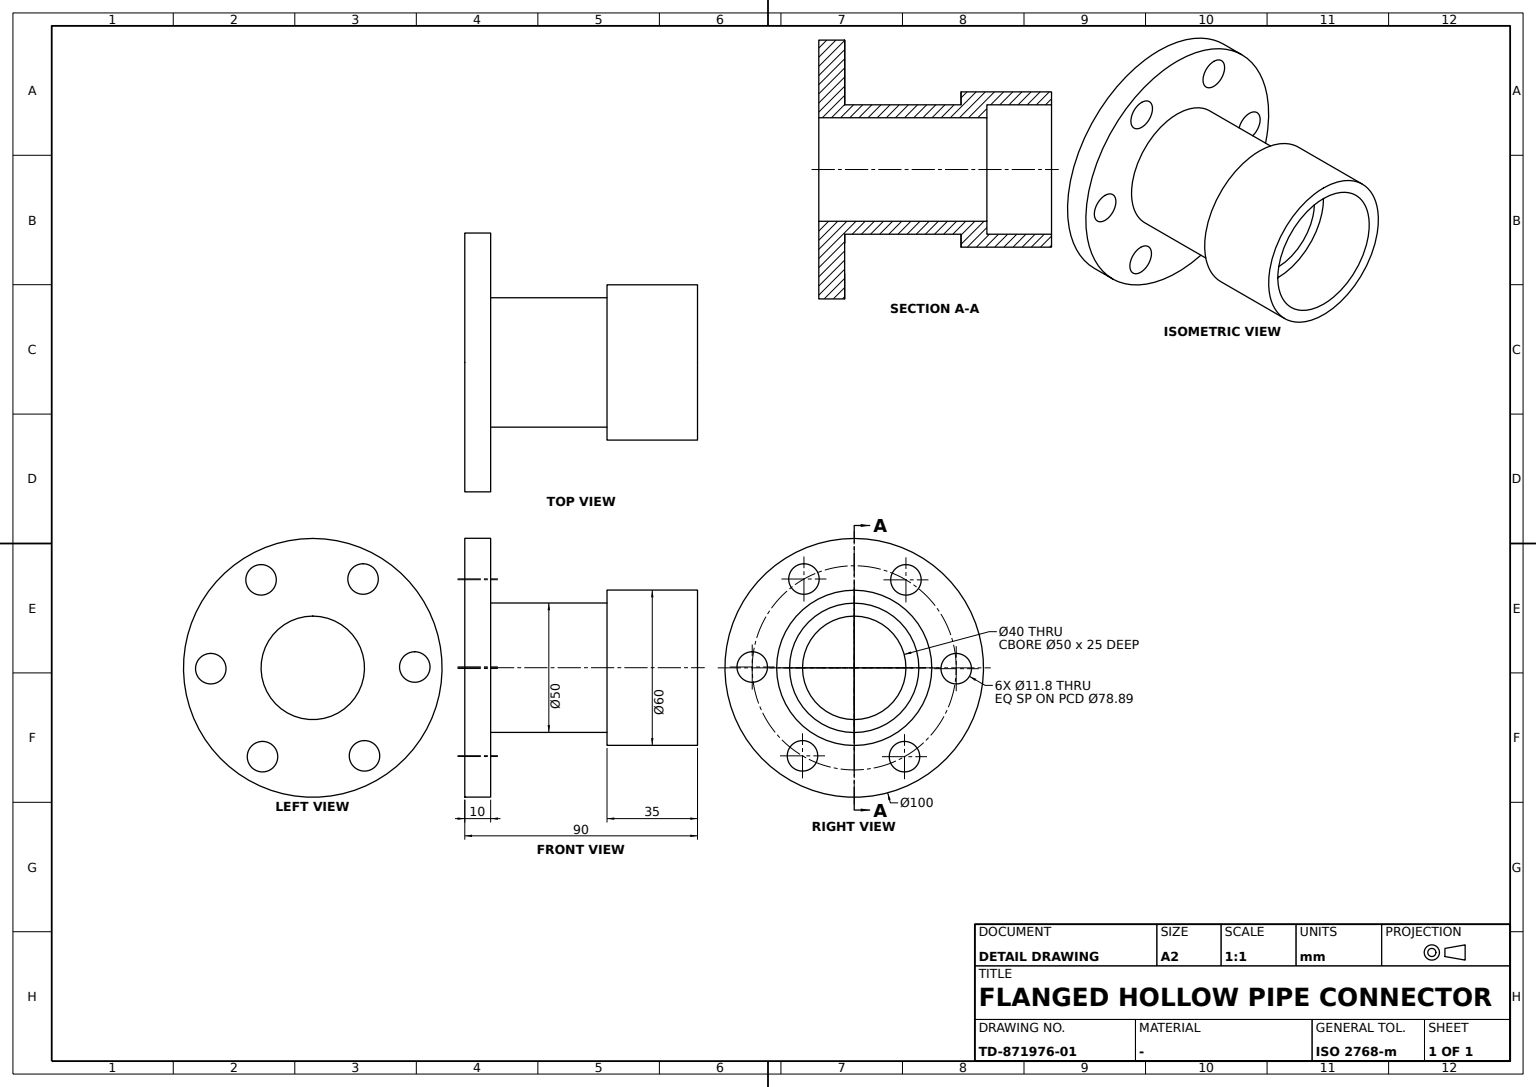
ISO-10303-21;
HEADER;
FILE_DESCRIPTION((''),'2;1');
FILE_NAME('','',(''),(''),'','','');
FILE_SCHEMA(('AUTOMOTIVE_DESIGN'));
ENDSEC;
DATA;
#1=APPLICATION_CONTEXT('');
#2=PRODUCT_CONTEXT('',#1,'mechanical');
#3=PRODUCT('','','',(#2));
#4=PRODUCT_DEFINITION_FORMATION('','',#3);
#5=PRODUCT_DEFINITION_CONTEXT('',#1,'design');
#6=PRODUCT_DEFINITION('','',#4,#5);
#7=PRODUCT_DEFINITION_SHAPE('','',#6);
#8=(LENGTH_UNIT()NAMED_UNIT(*)SI_UNIT(.MILLI.,.METRE.));
#9=(NAMED_UNIT(*)PLANE_ANGLE_UNIT()SI_UNIT($,.RADIAN.));
#10=(NAMED_UNIT(*)SI_UNIT($,.STERADIAN.)SOLID_ANGLE_UNIT());
#11=UNCERTAINTY_MEASURE_WITH_UNIT(LENGTH_MEASURE(0.005),#8,'distance_accuracy_value','');
#12=(GEOMETRIC_REPRESENTATION_CONTEXT(3)GLOBAL_UNCERTAINTY_ASSIGNED_CONTEXT((#11))GLOBAL_UNIT_ASSIGNED_CONTEXT((#8,#9,#10))REPRESENTATION_CONTEXT('',''));
#13=CARTESIAN_POINT('',(-35.,0.,25.));
#14=VERTEX_POINT('',#13);
#15=CARTESIAN_POINT('',(-35.,0.,0.));
#16=DIRECTION('',(-1.,0.,0.));
#17=DIRECTION('',(0.,0.,1.));
#18=AXIS2_PLACEMENT_3D('',#15,#16,#17);
#19=CIRCLE('',#18,25.);
#20=EDGE_CURVE('',#14,#14,#19,.T.);
#21=ORIENTED_EDGE('',*,*,#20,.F.);
#22=EDGE_LOOP('',(#21));
#23=FACE_BOUND('',#22,.T.);
#24=CARTESIAN_POINT('',(10.,0.,25.));
#25=VERTEX_POINT('',#24);
#26=CARTESIAN_POINT('',(10.,0.,0.));
#27=AXIS2_PLACEMENT_3D('',#26,#16,#17);
#28=CIRCLE('',#27,25.);
#29=EDGE_CURVE('',#25,#25,#28,.T.);
#30=ORIENTED_EDGE('',*,*,#29,.T.);
#31=EDGE_LOOP('',(#30));
#32=FACE_BOUND('',#31,.T.);
#33=CARTESIAN_POINT('',(0.,0.,0.));
#34=DIRECTION('',(0.,1.,0.));
#35=AXIS2_PLACEMENT_3D('',#33,#16,#34);
#36=CYLINDRICAL_SURFACE('',#35,25.);
#37=ADVANCED_FACE('',(#23,#32),#36,.T.);
#38=CARTESIAN_POINT('',(20.,0.,-20.));
#39=VERTEX_POINT('',#38);
#40=CARTESIAN_POINT('',(20.,0.,0.));
#41=DIRECTION('',(1.,0.,0.));
#42=DIRECTION('',(0.,0.,-1.));
#43=AXIS2_PLACEMENT_3D('',#40,#41,#42);
#44=CIRCLE('',#43,20.);
#45=EDGE_CURVE('',#39,#39,#44,.T.);
#46=ORIENTED_EDGE('',*,*,#45,.T.);
#47=EDGE_LOOP('',(#46));
#48=FACE_BOUND('',#47,.T.);
#49=CARTESIAN_POINT('',(-45.,0.,20.));
#50=VERTEX_POINT('',#49);
#51=CARTESIAN_POINT('',(-45.,0.,0.));
#52=AXIS2_PLACEMENT_3D('',#51,#16,#17);
#53=CIRCLE('',#52,20.);
#54=EDGE_CURVE('',#50,#50,#53,.F.);
#55=ORIENTED_EDGE('',*,*,#54,.F.);
#56=EDGE_LOOP('',(#55));
#57=FACE_BOUND('',#56,.T.);
#58=CARTESIAN_POINT('',(-12.5,0.,0.));
#59=AXIS2_PLACEMENT_3D('',#58,#41,#34);
#60=CYLINDRICAL_SURFACE('',#59,20.);
#61=ADVANCED_FACE('',(#48,#57),#60,.F.);
#62=CARTESIAN_POINT('',(-45.,19.444864,-28.420508));
#63=VERTEX_POINT('',#62);
#64=CARTESIAN_POINT('',(-45.,19.444864,-34.320508));
#65=AXIS2_PLACEMENT_3D('',#64,#16,#17);
#66=CIRCLE('',#65,5.9);
#67=EDGE_CURVE('',#63,#63,#66,.T.);
#68=ORIENTED_EDGE('',*,*,#67,.T.);
#69=EDGE_LOOP('',(#68));
#70=FACE_BOUND('',#69,.T.);
#71=CARTESIAN_POINT('',(-35.,19.444864,-28.420508));
#72=VERTEX_POINT('',#71);
#73=CARTESIAN_POINT('',(-35.,19.444864,-34.320508));
#74=AXIS2_PLACEMENT_3D('',#73,#16,#17);
#75=CIRCLE('',#74,5.9);
#76=EDGE_CURVE('',#72,#72,#75,.F.);
#77=ORIENTED_EDGE('',*,*,#76,.T.);
#78=EDGE_LOOP('',(#77));
#79=FACE_BOUND('',#78,.T.);
#80=CARTESIAN_POINT('',(-67.5,19.444864,-34.320508));
#81=DIRECTION('',(0.,-0.5,-0.866025404));
#82=AXIS2_PLACEMENT_3D('',#80,#41,#81);
#83=CYLINDRICAL_SURFACE('',#82,5.9);
#84=ADVANCED_FACE('',(#70,#79),#83,.F.);
#85=CARTESIAN_POINT('',(-45.,20.,39.9));
#86=VERTEX_POINT('',#85);
#87=CARTESIAN_POINT('',(-45.,20.,34.));
#88=AXIS2_PLACEMENT_3D('',#87,#16,#17);
#89=CIRCLE('',#88,5.9);
#90=EDGE_CURVE('',#86,#86,#89,.T.);
#91=ORIENTED_EDGE('',*,*,#90,.T.);
#92=EDGE_LOOP('',(#91));
#93=FACE_BOUND('',#92,.T.);
#94=CARTESIAN_POINT('',(-35.,20.,39.9));
#95=VERTEX_POINT('',#94);
#96=CARTESIAN_POINT('',(-35.,20.,34.));
#97=AXIS2_PLACEMENT_3D('',#96,#16,#17);
#98=CIRCLE('',#97,5.9);
#99=EDGE_CURVE('',#95,#95,#98,.F.);
#100=ORIENTED_EDGE('',*,*,#99,.T.);
#101=EDGE_LOOP('',(#100));
#102=FACE_BOUND('',#101,.T.);
#103=CARTESIAN_POINT('',(-67.5,20.,34.));
#104=AXIS2_PLACEMENT_3D('',#103,#41,#34);
#105=CYLINDRICAL_SURFACE('',#104,5.9);
#106=ADVANCED_FACE('',(#93,#102),#105,.F.);
#107=CARTESIAN_POINT('',(-35.,39.444864,5.579492));
#108=VERTEX_POINT('',#107);
#109=CARTESIAN_POINT('',(-35.,39.444864,-0.320508));
#110=AXIS2_PLACEMENT_3D('',#109,#16,#17);
#111=CIRCLE('',#110,5.9);
#112=EDGE_CURVE('',#108,#108,#111,.F.);
#113=ORIENTED_EDGE('',*,*,#112,.T.);
#114=EDGE_LOOP('',(#113));
#115=FACE_BOUND('',#114,.T.);
#116=CARTESIAN_POINT('',(-45.,39.444864,5.579492));
#117=VERTEX_POINT('',#116);
#118=CARTESIAN_POINT('',(-45.,39.444864,-0.320508));
#119=AXIS2_PLACEMENT_3D('',#118,#16,#17);
#120=CIRCLE('',#119,5.9);
#121=EDGE_CURVE('',#117,#117,#120,.T.);
#122=ORIENTED_EDGE('',*,*,#121,.T.);
#123=EDGE_LOOP('',(#122));
#124=FACE_BOUND('',#123,.T.);
#125=CARTESIAN_POINT('',(-67.5,39.444864,-0.320508));
#126=DIRECTION('',(0.,0.5,-0.866025404));
#127=AXIS2_PLACEMENT_3D('',#125,#41,#126);
#128=CYLINDRICAL_SURFACE('',#127,5.9);
#129=ADVANCED_FACE('',(#115,#124),#128,.F.);
#130=CARTESIAN_POINT('',(45.,0.,30.));
#131=VERTEX_POINT('',#130);
#132=CARTESIAN_POINT('',(45.,0.,0.));
#133=AXIS2_PLACEMENT_3D('',#132,#16,#17);
#134=CIRCLE('',#133,30.);
#135=EDGE_CURVE('',#131,#131,#134,.T.);
#136=ORIENTED_EDGE('',*,*,#135,.T.);
#137=EDGE_LOOP('',(#136));
#138=FACE_BOUND('',#137,.T.);
#139=CARTESIAN_POINT('',(10.,0.,30.));
#140=VERTEX_POINT('',#139);
#141=CIRCLE('',#27,30.);
#142=EDGE_CURVE('',#140,#140,#141,.T.);
#143=ORIENTED_EDGE('',*,*,#142,.F.);
#144=EDGE_LOOP('',(#143));
#145=FACE_BOUND('',#144,.T.);
#146=CYLINDRICAL_SURFACE('',#35,30.);
#147=ADVANCED_FACE('',(#138,#145),#146,.T.);
#148=CARTESIAN_POINT('',(-45.,-39.444864,6.220508));
#149=VERTEX_POINT('',#148);
#150=CARTESIAN_POINT('',(-45.,-39.444864,0.320508));
#151=AXIS2_PLACEMENT_3D('',#150,#16,#17);
#152=CIRCLE('',#151,5.9);
#153=EDGE_CURVE('',#149,#149,#152,.T.);
#154=ORIENTED_EDGE('',*,*,#153,.T.);
#155=EDGE_LOOP('',(#154));
#156=FACE_BOUND('',#155,.T.);
#157=CARTESIAN_POINT('',(-35.,-39.444864,6.220508));
#158=VERTEX_POINT('',#157);
#159=CARTESIAN_POINT('',(-35.,-39.444864,0.320508));
#160=AXIS2_PLACEMENT_3D('',#159,#16,#17);
#161=CIRCLE('',#160,5.9);
#162=EDGE_CURVE('',#158,#158,#161,.F.);
#163=ORIENTED_EDGE('',*,*,#162,.T.);
#164=EDGE_LOOP('',(#163));
#165=FACE_BOUND('',#164,.T.);
#166=CARTESIAN_POINT('',(-67.5,-39.444864,0.320508));
#167=DIRECTION('',(0.,-0.5,0.866025404));
#168=AXIS2_PLACEMENT_3D('',#166,#41,#167);
#169=CYLINDRICAL_SURFACE('',#168,5.9);
#170=ADVANCED_FACE('',(#156,#165),#169,.F.);
#171=CARTESIAN_POINT('',(20.,0.,-25.));
#172=VERTEX_POINT('',#171);
#173=CIRCLE('',#43,25.);
#174=EDGE_CURVE('',#172,#172,#173,.T.);
#175=ORIENTED_EDGE('',*,*,#174,.T.);
#176=EDGE_LOOP('',(#175));
#177=FACE_BOUND('',#176,.T.);
#178=ORIENTED_EDGE('',*,*,#45,.F.);
#179=EDGE_LOOP('',(#178));
#180=FACE_BOUND('',#179,.T.);
#181=AXIS2_PLACEMENT_3D('',#40,#41,#34);
#182=PLANE('',#181);
#183=ADVANCED_FACE('',(#177,#180),#182,.T.);
#184=CARTESIAN_POINT('',(45.,0.,25.));
#185=VERTEX_POINT('',#184);
#186=CIRCLE('',#133,25.);
#187=EDGE_CURVE('',#185,#185,#186,.F.);
#188=ORIENTED_EDGE('',*,*,#187,.T.);
#189=EDGE_LOOP('',(#188));
#190=FACE_BOUND('',#189,.T.);
#191=ORIENTED_EDGE('',*,*,#174,.F.);
#192=EDGE_LOOP('',(#191));
#193=FACE_BOUND('',#192,.T.);
#194=ADVANCED_FACE('',(#190,#193),#36,.F.);
#195=ORIENTED_EDGE('',*,*,#112,.F.);
#196=EDGE_LOOP('',(#195));
#197=FACE_BOUND('',#196,.T.);
#198=ORIENTED_EDGE('',*,*,#20,.T.);
#199=EDGE_LOOP('',(#198));
#200=FACE_BOUND('',#199,.T.);
#201=ORIENTED_EDGE('',*,*,#99,.F.);
#202=EDGE_LOOP('',(#201));
#203=FACE_BOUND('',#202,.T.);
#204=CARTESIAN_POINT('',(-35.,-19.444864,40.220508));
#205=VERTEX_POINT('',#204);
#206=CARTESIAN_POINT('',(-35.,-19.444864,34.320508));
#207=AXIS2_PLACEMENT_3D('',#206,#16,#17);
#208=CIRCLE('',#207,5.9);
#209=EDGE_CURVE('',#205,#205,#208,.F.);
#210=ORIENTED_EDGE('',*,*,#209,.F.);
#211=EDGE_LOOP('',(#210));
#212=FACE_BOUND('',#211,.T.);
#213=ORIENTED_EDGE('',*,*,#162,.F.);
#214=EDGE_LOOP('',(#213));
#215=FACE_BOUND('',#214,.T.);
#216=CARTESIAN_POINT('',(-35.,-20.,-28.1));
#217=VERTEX_POINT('',#216);
#218=CARTESIAN_POINT('',(-35.,-20.,-34.));
#219=AXIS2_PLACEMENT_3D('',#218,#16,#17);
#220=CIRCLE('',#219,5.9);
#221=EDGE_CURVE('',#217,#217,#220,.F.);
#222=ORIENTED_EDGE('',*,*,#221,.F.);
#223=EDGE_LOOP('',(#222));
#224=FACE_BOUND('',#223,.T.);
#225=CARTESIAN_POINT('',(-35.,0.,50.));
#226=VERTEX_POINT('',#225);
#227=CIRCLE('',#18,50.);
#228=EDGE_CURVE('',#226,#226,#227,.T.);
#229=ORIENTED_EDGE('',*,*,#228,.F.);
#230=EDGE_LOOP('',(#229));
#231=FACE_BOUND('',#230,.T.);
#232=ORIENTED_EDGE('',*,*,#76,.F.);
#233=EDGE_LOOP('',(#232));
#234=FACE_BOUND('',#233,.T.);
#235=AXIS2_PLACEMENT_3D('',#13,#16,#34);
#236=PLANE('',#235);
#237=ADVANCED_FACE('',(#197,#200,#203,#212,#215,#224,#231,#234),#236,.F.);
#238=ORIENTED_EDGE('',*,*,#135,.F.);
#239=EDGE_LOOP('',(#238));
#240=FACE_BOUND('',#239,.T.);
#241=ORIENTED_EDGE('',*,*,#187,.F.);
#242=EDGE_LOOP('',(#241));
#243=FACE_BOUND('',#242,.T.);
#244=AXIS2_PLACEMENT_3D('',#132,#16,#34);
#245=PLANE('',#244);
#246=ADVANCED_FACE('',(#240,#243),#245,.F.);
#247=ORIENTED_EDGE('',*,*,#209,.T.);
#248=EDGE_LOOP('',(#247));
#249=FACE_BOUND('',#248,.T.);
#250=CARTESIAN_POINT('',(-45.,-19.444864,40.220508));
#251=VERTEX_POINT('',#250);
#252=CARTESIAN_POINT('',(-45.,-19.444864,34.320508));
#253=AXIS2_PLACEMENT_3D('',#252,#16,#17);
#254=CIRCLE('',#253,5.9);
#255=EDGE_CURVE('',#251,#251,#254,.T.);
#256=ORIENTED_EDGE('',*,*,#255,.T.);
#257=EDGE_LOOP('',(#256));
#258=FACE_BOUND('',#257,.T.);
#259=CARTESIAN_POINT('',(-67.5,-19.444864,34.320508));
#260=DIRECTION('',(0.,0.5,0.866025404));
#261=AXIS2_PLACEMENT_3D('',#259,#41,#260);
#262=CYLINDRICAL_SURFACE('',#261,5.9);
#263=ADVANCED_FACE('',(#249,#258),#262,.F.);
#264=ORIENTED_EDGE('',*,*,#29,.F.);
#265=EDGE_LOOP('',(#264));
#266=FACE_BOUND('',#265,.T.);
#267=ORIENTED_EDGE('',*,*,#142,.T.);
#268=EDGE_LOOP('',(#267));
#269=FACE_BOUND('',#268,.T.);
#270=AXIS2_PLACEMENT_3D('',#139,#16,#34);
#271=PLANE('',#270);
#272=ADVANCED_FACE('',(#266,#269),#271,.T.);
#273=ORIENTED_EDGE('',*,*,#228,.T.);
#274=EDGE_LOOP('',(#273));
#275=FACE_BOUND('',#274,.T.);
#276=CARTESIAN_POINT('',(-45.,0.,50.));
#277=VERTEX_POINT('',#276);
#278=CIRCLE('',#52,50.);
#279=EDGE_CURVE('',#277,#277,#278,.T.);
#280=ORIENTED_EDGE('',*,*,#279,.F.);
#281=EDGE_LOOP('',(#280));
#282=FACE_BOUND('',#281,.T.);
#283=CYLINDRICAL_SURFACE('',#35,50.);
#284=ADVANCED_FACE('',(#275,#282),#283,.T.);
#285=ORIENTED_EDGE('',*,*,#279,.T.);
#286=EDGE_LOOP('',(#285));
#287=FACE_BOUND('',#286,.T.);
#288=ORIENTED_EDGE('',*,*,#90,.F.);
#289=EDGE_LOOP('',(#288));
#290=FACE_BOUND('',#289,.T.);
#291=CARTESIAN_POINT('',(-45.,-20.,-28.1));
#292=VERTEX_POINT('',#291);
#293=CARTESIAN_POINT('',(-45.,-20.,-34.));
#294=AXIS2_PLACEMENT_3D('',#293,#16,#17);
#295=CIRCLE('',#294,5.9);
#296=EDGE_CURVE('',#292,#292,#295,.T.);
#297=ORIENTED_EDGE('',*,*,#296,.F.);
#298=EDGE_LOOP('',(#297));
#299=FACE_BOUND('',#298,.T.);
#300=ORIENTED_EDGE('',*,*,#67,.F.);
#301=EDGE_LOOP('',(#300));
#302=FACE_BOUND('',#301,.T.);
#303=ORIENTED_EDGE('',*,*,#153,.F.);
#304=EDGE_LOOP('',(#303));
#305=FACE_BOUND('',#304,.T.);
#306=ORIENTED_EDGE('',*,*,#54,.T.);
#307=EDGE_LOOP('',(#306));
#308=FACE_BOUND('',#307,.T.);
#309=ORIENTED_EDGE('',*,*,#255,.F.);
#310=EDGE_LOOP('',(#309));
#311=FACE_BOUND('',#310,.T.);
#312=ORIENTED_EDGE('',*,*,#121,.F.);
#313=EDGE_LOOP('',(#312));
#314=FACE_BOUND('',#313,.T.);
#315=AXIS2_PLACEMENT_3D('',#276,#16,#34);
#316=PLANE('',#315);
#317=ADVANCED_FACE('',(#287,#290,#299,#302,#305,#308,#311,#314),#316,.T.);
#318=ORIENTED_EDGE('',*,*,#296,.T.);
#319=EDGE_LOOP('',(#318));
#320=FACE_BOUND('',#319,.T.);
#321=ORIENTED_EDGE('',*,*,#221,.T.);
#322=EDGE_LOOP('',(#321));
#323=FACE_BOUND('',#322,.T.);
#324=CARTESIAN_POINT('',(-67.5,-20.,-34.));
#325=DIRECTION('',(0.,-1.,0.));
#326=AXIS2_PLACEMENT_3D('',#324,#41,#325);
#327=CYLINDRICAL_SURFACE('',#326,5.9);
#328=ADVANCED_FACE('',(#320,#323),#327,.F.);
#329=CLOSED_SHELL('',(#37,#61,#84,#106,#129,#147,#170,#183,#194,#237,#246,#263,#272,#284,#317,#328));
#330=MANIFOLD_SOLID_BREP('',#329);
#331=ADVANCED_BREP_SHAPE_REPRESENTATION('',(#330),#12);
#332=SHAPE_DEFINITION_REPRESENTATION(#7,#331);
ENDSEC;
END-ISO-10303-21;
